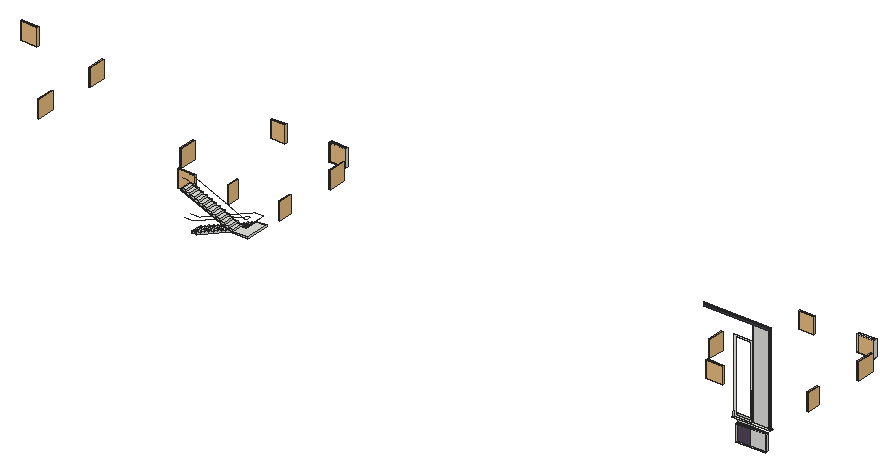
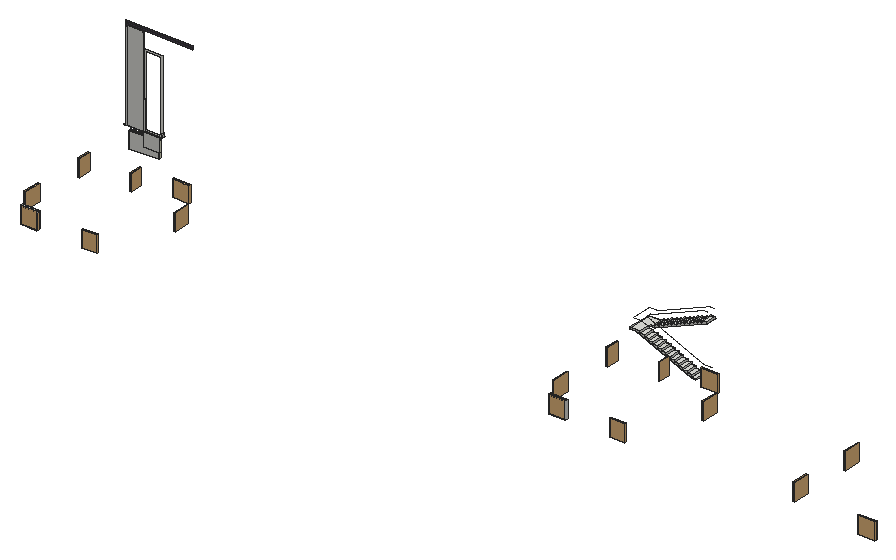
# SketchUp Ruby script. Lengths in inches.
U = 1.inch
M = Sketchup.active_model
def pt(a) = Geom::Point3d.new(a.map { |v| v * U })
def face(e, loops, mat)
  f = e.add_face(loops[0].map { |a| pt(a) })
  loops[1..].each { |l| e.add_face(l.map { |a| pt(a) }).erase! }
  f.material = f.back_material = mat if mat
  f
end
# faces: each face lists its corners as indices into pts; further lists are holes
def faces(e, pts, list, mat = nil) = list.each { |f| face(e, (f[0].is_a?(Array) ? f : [f]).map { |l| l.map { |i| pts[i] } }, mat) }
# xy, xz, yz: faces in a plane at the given z, y or x. An outline is a flat list of corners, or four numbers for a rectangle; further outlines are holes
def ring(l) = l.size == 4 ? [[l[0], l[1]], [l[2], l[1]], [l[2], l[3]], [l[0], l[3]]] : l.each_slice(2).to_a
def flat(e, list, mat, &to3) = list.each { |f| face(e, (f[0].is_a?(Array) ? f : [f]).map { |l| ring(l).map { |u, v| to3.(u, v) } }, mat) }
def xy(e, z, list, mat = nil) = flat(e, list, mat) { |x, y| [x, y, z] }
def xz(e, y, list, mat = nil) = flat(e, list, mat) { |x, z| [x, y, z] }
def yz(e, x, list, mat = nil) = flat(e, list, mat) { |y, z| [x, y, z] }
def lines(e, pts, list) = list.each { |a, b| e.add_line(pt(pts[a]), pt(pts[b])) }
# prism: a flat outline (further loops are holes) pulled along v
def prism(e, loops, v, mat = nil)
  f = face(e, loops, mat); d = Geom::Vector3d.new(v.map { |x| x * U })
  f.pushpull(f.normal.samedirection?(d) ? d.length : -d.length)
end
def box(e, o, s, mat = nil) = prism(e, [[o, [o[0] + s[0], o[1], o[2]], [o[0] + s[0], o[1] + s[1], o[2]], [o[0], o[1] + s[1], o[2]]]], [0, 0, s[2]], mat)
def at(x, y, z, deg = 0) = Geom::Transformation.translation(pt([x, y, z])) * Geom::Transformation.rotation(ORIGIN, Z_AXIS, deg.degrees)
def axes(o, x, y, z) = Geom::Transformation.new([*x, 0, *y, 0, *z, 0, *pt(o).to_a, 1])
def part(name) = M.definitions.add(name)
# library, detail: a bought-in or finely detailed component or shape, given as its bounding box
def library(name, o, s) = part(name).tap { |d| box(d.entities, o, s) }
def detail(e, o, s) = box(e.add_group.entities, o, s)
def put(e, d, t, mat = nil) = e.add_instance(d, t).tap { |i| i.material = mat if mat }
def group(e, t, mat = nil) = e.add_group.tap { |g| g.transformation = t; g.material = mat if mat }.entities
root = M.entities
M.materials.add("0113 AP L161 ABSOLUTE WHITE").color = [243, 242, 236]
M.materials.add("0280 AP 9627 Emperor_s Purple-N").color = [83, 70, 91]
M.materials.add("0746 AP 7715 LUMINOUS").color = [235, 235, 209]
M.materials.add("M00_Soft_Cloud").color = [255, 255, 255]
c1 = part("Group19\#2")
p = [[1706.5625,247.76,0],[1706.5625,271.76,0],[1706.5625,427.76,65],[1706.5625,431.76,65],[1720.5625,431.76,65],[1720.5625,427.76,65],
  [1720.5625,283.76,125],[1720.5625,271.76,125],[1686.5625,247.76,0],[1686.5625,271.76,0],[1686.5625,427.76,65],[1686.5625,451.76,65],
  [1740.5625,451.76,65],[1740.5625,427.76,65],[1740.5625,283.76,125],[1740.5625,271.76,125]]
lines(c1.entities,p,[[0,1],[1,2],[2,3],[3,4],[4,5],[5,6],[6,7],[8,9],[9,10],[10,11],[11,12],[12,13],
  [13,14],[14,15]])
c2 = part("Group18\#3")
xy(c2.entities,-3.9375,[[1682.5625,271.76,1710.5625,283.76],[1682.5625,283.76,1710.5625,284.55]])
xy(c2.entities,0,[[1682.5625,271.76,1710.5625,283.76]])
xy(c2.entities,5,[[1682.5625,283.76,1710.5625,295.76]])
xy(c2.entities,10,[[1682.5625,295.76,1710.5625,307.76]])
xy(c2.entities,15,[[1682.5625,307.76,1710.5625,319.76]])
xy(c2.entities,20,[[1682.5625,319.76,1710.5625,331.76]])
xy(c2.entities,25,[[1682.5625,331.76,1710.5625,343.76]])
xy(c2.entities,30,[[1682.5625,343.76,1710.5625,355.76]])
xy(c2.entities,35,[[1682.5625,355.76,1710.5625,367.76]])
xy(c2.entities,40,[[1682.5625,367.76,1710.5625,379.76]])
xy(c2.entities,45,[[1682.5625,379.76,1710.5625,391.76]])
xy(c2.entities,50,[[1682.5625,391.76,1710.5625,403.76]])
xy(c2.entities,55,[[1682.5625,403.76,1710.5625,415.76]])
xy(c2.entities,60,[[1682.5625,415.76,1710.5625,427.76]])
xy(c2.entities,61.0625,[[1716.5625,414.97,1716.5625,427.76,1710.5625,427.76,1710.5625,440.55,1682.5625,440.55,1682.5625,455.76,1744.5625,455.76,1744.5625,414.97]])
xy(c2.entities,65,[[1716.5625,415.76,1744.5625,415.76,1744.5625,455.76,1682.5625,455.76,1682.5625,427.76,1716.5625,427.76]])
xy(c2.entities,70,[[1716.5625,403.76,1744.5625,415.76]])
xy(c2.entities,75,[[1716.5625,391.76,1744.5625,403.76]])
xy(c2.entities,80,[[1716.5625,379.76,1744.5625,391.76]])
xy(c2.entities,85,[[1716.5625,367.76,1744.5625,379.76]])
xy(c2.entities,90,[[1716.5625,355.76,1744.5625,367.76]])
xy(c2.entities,95,[[1716.5625,343.76,1744.5625,355.76]])
xy(c2.entities,100,[[1716.5625,331.76,1744.5625,343.76]])
xy(c2.entities,105,[[1716.5625,319.76,1744.5625,331.76]])
xy(c2.entities,110,[[1716.5625,307.76,1744.5625,319.76]])
xy(c2.entities,115,[[1716.5625,295.76,1744.5625,307.76]])
xy(c2.entities,120,[[1716.5625,283.76,1744.5625,295.76]])
xy(c2.entities,121.0625,[[1716.5625,270.97,1744.5625,271.76]])
xy(c2.entities,125,[[1716.5625,271.76,1744.5625,283.76]])
xz(c2.entities,271.76,[[1682.5625,-3.9375,1710.5625,0],[1716.5625,121.0625,1744.5625,125]])
xz(c2.entities,283.76,[[1682.5625,-3.9375,1710.5625,0],[1682.5625,0,1710.5625,5],[1716.5625,120,1744.5625,125]])
xz(c2.entities,295.76,[[1682.5625,5,1710.5625,10],[1716.5625,115,1744.5625,120]])
xz(c2.entities,307.76,[[1682.5625,10,1710.5625,15],[1716.5625,110,1744.5625,115]])
xz(c2.entities,319.76,[[1682.5625,15,1710.5625,20],[1716.5625,105,1744.5625,110]])
xz(c2.entities,331.76,[[1682.5625,20,1710.5625,25],[1716.5625,100,1744.5625,105]])
xz(c2.entities,343.76,[[1682.5625,25,1710.5625,30],[1716.5625,95,1744.5625,100]])
xz(c2.entities,355.76,[[1682.5625,30,1710.5625,35],[1716.5625,90,1744.5625,95]])
xz(c2.entities,367.76,[[1682.5625,35,1710.5625,40],[1716.5625,85,1744.5625,90]])
xz(c2.entities,379.76,[[1682.5625,40,1710.5625,45],[1716.5625,80,1744.5625,85]])
xz(c2.entities,391.76,[[1682.5625,45,1710.5625,50],[1716.5625,75,1744.5625,80]])
xz(c2.entities,403.76,[[1682.5625,50,1710.5625,55],[1716.5625,70,1744.5625,75]])
xz(c2.entities,415.76,[[1682.5625,55,1710.5625,60],[1716.5625,65,1744.5625,70]])
xz(c2.entities,427.76,[[1682.5625,60,1710.5625,65],[1710.5625,61.0625,1716.5625,65]])
xz(c2.entities,455.76,[[1682.5625,61.0625,1744.5625,65]])
yz(c2.entities,1682.5625,[[271.76,-3.9375,283.76,0],[283.76,-3.9375,283.76,5,295.76,5,295.76,10,307.76,10,307.76,15,319.76,15,319.76,20,331.76,20,331.76,25,343.76,25,343.76,30,355.76,30,355.76,35,367.76,35,367.76,40,379.76,40,379.76,45,391.76,45,391.76,50,403.76,50,403.76,55,415.76,55,415.76,60,427.76,60,427.76,65,455.76,65,455.76,61.0625,440.55,61.0625,284.55,-3.9375]])
yz(c2.entities,1710.5625,[[271.76,-3.9375,283.76,0],[283.76,-3.9375,284.55,-3.9375,440.55,61.0625,427.76,61.0625,427.76,60,415.76,60,415.76,55,403.76,55,403.76,50,391.76,50,391.76,45,379.76,45,379.76,40,367.76,40,367.76,35,355.76,35,355.76,30,343.76,30,343.76,25,331.76,25,331.76,20,319.76,20,319.76,15,307.76,15,307.76,10,295.76,10,295.76,5,283.76,5]])
yz(c2.entities,1716.5625,[[414.97,61.0625,270.97,121.0625,271.76,121.0625,271.76,125,283.76,125,283.76,120,295.76,120,295.76,115,307.76,115,307.76,110,319.76,110,319.76,105,331.76,105,331.76,100,343.76,100,343.76,95,355.76,95,355.76,90,367.76,90,367.76,85,379.76,85,379.76,80,391.76,80,391.76,75,403.76,75,403.76,70,415.76,70,415.76,65,427.76,65,427.76,61.0625]])
yz(c2.entities,1744.5625,[[414.97,61.0625,455.76,61.0625,455.76,65,415.76,65,415.76,70,403.76,70,403.76,75,391.76,75,391.76,80,379.76,80,379.76,85,367.76,85,367.76,90,355.76,90,355.76,95,343.76,95,343.76,100,331.76,100,331.76,105,319.76,105,319.76,110,307.76,110,307.76,115,295.76,115,295.76,120,283.76,120,283.76,125,271.76,125,271.76,121.0625,270.97,121.0625]])
p = [[1682.5625,284.55,-3.9375],[1682.5625,440.55,61.0625],[1710.5625,440.55,61.0625],[1710.5625,284.55,-3.9375],[1744.5625,414.97,61.0625],[1744.5625,270.97,121.0625],
  [1716.5625,270.97,121.0625],[1716.5625,414.97,61.0625]]
faces(c2.entities,p,[[0,1,2,3],[4,5,6,7]])
put(c2.entities,c1,at(0,0,24))
c3 = library("Slide Window 5'",[0,-2.02,0],[60,2.02,54])
xy(root,11.32,[[2460.81,103.82,2499.73,105.28,2543.1,106.92,2542.91,111.91,2460.625,108.82]])
xy(root,11.32,[[2460.97,99.82,2543.25,102.92,2543.1,106.92,2499.73,105.28,2460.81,103.82]],"0746 AP 7715 LUMINOUS")
xy(root,34.24,[[2443.89,551.55,2491.34,560.54]])
xy(root,36,[[991.15,491.43,1038.6,500.42]])
xy(root,57.55,[[2460.81,103.82,2460.625,108.82,2499.54,110.28,2499.73,105.28],[2499.73,105.28,2499.54,110.28,2542.91,111.91,2543.1,106.92]])
xy(root,57.55,[[2460.97,99.82,2460.81,103.82,2499.73,105.28,2543.1,106.92,2543.25,102.92]],"0746 AP 7715 LUMINOUS")
xy(root,69.55,[[2448.6,103.36,2448.64,108.36],[2552.4,105.16,2552.4,105.36,2549.9,105.36,2549.9,112.18,2554.91,112.36,2554.91,105.36,2553.2,105.36,2553.2,105.16],[2448.6,108.36,2448.64,112.36],[2448.64,108.36,2448.64,112.36,2499.54,112.36,2499.54,110.28],[2448.64,108.36,2499.54,108.36,2499.54,110.28],
  [2549.9,112.18,2549.9,112.36,2554.91,112.36]])
xy(root,69.55,[[2448.97,99.37,2555.24,103.37,2554.91,112.36,2554.91,105.36,2553.2,105.36,2553.2,105.16,2552.4,105.16,2552.4,105.36,2549.9,105.36,2549.9,112.18,2499.54,110.28,2499.54,108.36,2448.64,108.36]],"0746 AP 7715 LUMINOUS")
xy(root,80.8,[[2443.89,551.55,2491.34,560.54]])
xy(root,84,[[991.15,491.43,1038.6,500.42]])
xz(root,105.16,[[2552.4,69.55,2553.2,69.55,2553.2,327.8,2366.69,327.8,2366.69,327,2552.4,327]],"M00_Soft_Cloud")
xz(root,105.36,[[2549.9,69.55,2552.4,69.55,2552.4,327,2366.69,327,2366.69,322.5,2549.9,322.5],[2553.2,69.55,2554.91,69.55,2554.91,331.5,2366.69,331.5,2366.69,327.8,2553.2,327.8]],"0280 AP 9627 Emperor_s Purple-N")
xz(root,108.36,[[[2448.6,69.55,2499.54,278.5],[2452.6,73.55,2495.6,274.5]]],"0113 AP L161 ABSOLUTE WHITE")
xz(root,112.36,[[2448.6,69.55,2448.64,80.8],[2549.9,69.55,2550.375,115.5]])
xz(root,117.37,[[2452.6,33.75,2495.6,73.55]])
yz(root,991.15,[[491.43,36,500.42,84]])
yz(root,1038.6,[[491.43,36,500.42,84]])
yz(root,2443.89,[[551.55,34.24,560.54,80.8]])
yz(root,2448.6,[[103.36,69.55,108.36,80.8],[108.36,69.55,112.36,80.8]])
yz(root,2491.34,[[551.55,34.24,560.54,80.8]])
yz(root,2499.54,[[108.36,69.55,112.36,151.5]])
yz(root,2549.9,[[105.36,69.55,112.36,322.5]],"0280 AP 9627 Emperor_s Purple-N")
yz(root,2552.4,[[105.16,69.55,105.36,327]])
yz(root,2553.2,[[105.16,69.55,105.36,327]])
p = [[2460.97,99.82,11.32],[2460.81,103.82,11.32],[2460.81,103.82,57.55],[2460.97,99.82,57.55],[2543.25,102.92,57.55],[2543.1,106.92,57.55],
  [2543.1,106.92,11.32],[2543.25,102.92,11.32],[2460.625,108.82,11.32],[2460.625,108.82,57.55],[2499.73,105.28,11.32],[2499.73,105.28,57.55],
  [2542.91,111.91,57.55],[2542.91,111.91,11.32],[2499.54,110.28,57.55],[2495.6,112.36,33.75],[2495.625,112.36,33.75],[2452.6,112.36,33.75],
  [2452.625,112.36,33.75],[2495.6,117.37,33.75],[2452.6,117.37,33.75]]
faces(root,p,[[0,1,2,3],[4,5,6,7]],"0746 AP 7715 LUMINOUS")
faces(root,p,[[8,9,2,1],[5,11,10,6],[12,13,6,5],[13,8,9,14,12]])
faces(root,p,[[1,10,11,2]],"0280 AP 9627 Emperor_s Purple-N")
lines(root,p,[[15,16],[17,18],[15,19],[17,20]])
put(root,c2,axes([624.89,1974.23,5.15],[0.01009,-1.09803,0],[1.00962,0.00928,0],[0,0,1.01]))
put(root,c3,axes([2526.125,313.12,33.7],[0,-0.616,0],[2.31,0,0],[0,0,0.87219]))
put(root,c3,axes([2526,503.55,33.77],[0,-0.8,0],[2.31,0,0],[0,0,0.87084]))
put(root,c3,axes([2276.88,558.29,34.24],[0.68602,0,0],[0,2.31,0],[0,0,0.8536]))
put(root,c3,axes([2443.89,558.29,34.24],[0.7908,0,0],[0,2.31,0],[0,0,0.86222]))
put(root,c3,axes([2255.59,255.18,34.24],[0.79445,0,0],[0,2.31,0],[0,0,0.86222]))
put(root,c3,axes([2201.39,326.74,34.24],[0,0.75429,0],[-2.31,0,0],[0,0,0.87219]))
put(root,c3,axes([2393.03,293.04,34.8125],[0,-0.53878,0],[2.31,0,0],[0,0,0.87219]))
put(root,c3,axes([1073.38,252.99,35.44],[0,-0.616,0],[2.31,0,0],[0,0,0.89917]))
put(root,c3,axes([1073.25,443.43,35.52],[0,-0.8,0],[2.31,0,0],[0,0,0.89778]))
put(root,c3,axes([367.63,471.95,35.52],[0,-0.8005,0],[2.31,0,0],[0,0,0.89771]))
put(root,c3,axes([367.47,290.45,35.94],[0,-0.80083,0],[2.31,0,0],[0,0,0.89771]))
put(root,c3,axes([824.14,498.17,36],[0.68602,0,0],[0,2.31,0],[0,0,0.88]))
put(root,c3,axes([991.15,498.17,36],[0.7908,0,0],[0,2.31,0],[0,0,0.88889]))
put(root,c3,axes([112.97,498.17,36],[0.79979,0,0],[0,2.31,0],[0,0,0.88889]))
put(root,c3,axes([802.84,195.06,36],[0.79445,0,0],[0,2.31,0],[0,0,0.88889]))
put(root,c3,axes([748.65,266.62,36],[0,0.75429,0],[-2.31,0,0],[0,0,0.89917]))
put(root,c3,axes([940.28,232.91,36.59],[0,-0.53878,0],[2.31,0,0],[0,0,0.89917]))
g1 = group(root,at(2499.98,112.36,272.26))
xy(g1,-202.71,[[0,-1.66,49.92,-0.6]])
xy(g1,50.23,[[0,-1.66,49.92,-0.6]])
xz(g1,-1.66,[[0,-202.71,49.92,50.23]])
yz(g1,0,[[-1.66,-202.71,-0.6,50.23]])
yz(g1,49.92,[[-1.66,-202.71,-0.6,50.23]])
